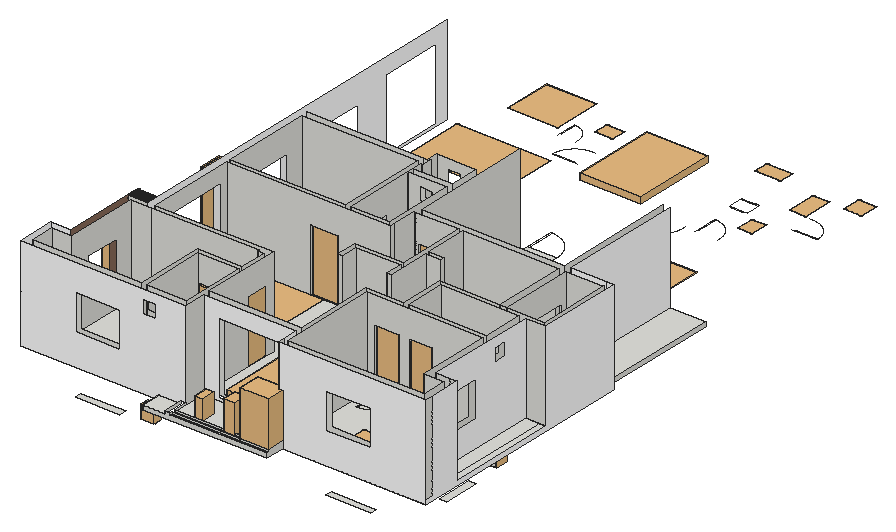
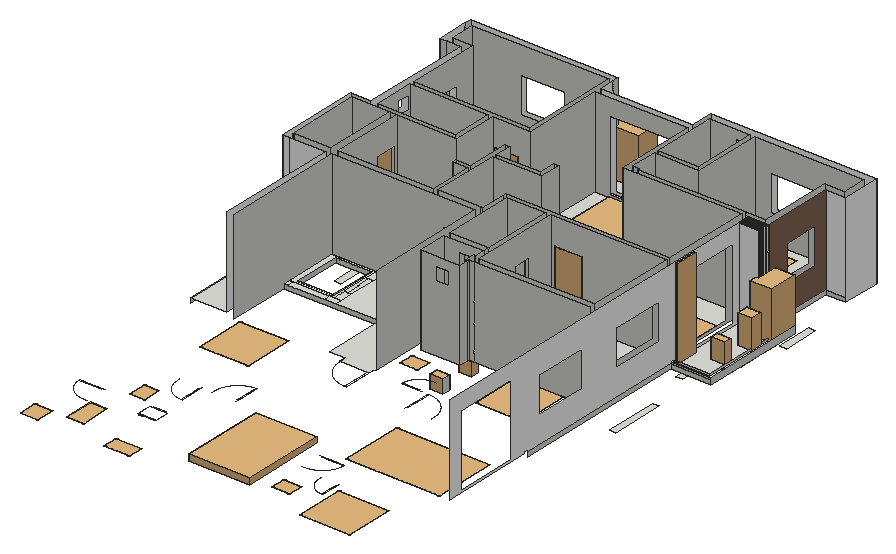
# SketchUp Ruby script. Lengths in inches.
U = 1.inch
M = Sketchup.active_model
def pt(a) = Geom::Point3d.new(a.map { |v| v * U })
def face(e, loops, mat)
  f = e.add_face(loops[0].map { |a| pt(a) })
  loops[1..].each { |l| e.add_face(l.map { |a| pt(a) }).erase! }
  f.material = f.back_material = mat if mat
  f
end
# faces: each face lists its corners as indices into pts; further lists are holes
def faces(e, pts, list, mat = nil) = list.each { |f| face(e, (f[0].is_a?(Array) ? f : [f]).map { |l| l.map { |i| pts[i] } }, mat) }
# xy, xz, yz: faces in a plane at the given z, y or x. An outline is a flat list of corners, or four numbers for a rectangle; further outlines are holes
def ring(l) = l.size == 4 ? [[l[0], l[1]], [l[2], l[1]], [l[2], l[3]], [l[0], l[3]]] : l.each_slice(2).to_a
def flat(e, list, mat, &to3) = list.each { |f| face(e, (f[0].is_a?(Array) ? f : [f]).map { |l| ring(l).map { |u, v| to3.(u, v) } }, mat) }
def xy(e, z, list, mat = nil) = flat(e, list, mat) { |x, y| [x, y, z] }
def xz(e, y, list, mat = nil) = flat(e, list, mat) { |x, z| [x, y, z] }
def yz(e, x, list, mat = nil) = flat(e, list, mat) { |y, z| [x, y, z] }
def lines(e, pts, list) = list.each { |a, b| e.add_line(pt(pts[a]), pt(pts[b])) }
# prism: a flat outline (further loops are holes) pulled along v
def prism(e, loops, v, mat = nil)
  f = face(e, loops, mat); d = Geom::Vector3d.new(v.map { |x| x * U })
  f.pushpull(f.normal.samedirection?(d) ? d.length : -d.length)
end
def box(e, o, s, mat = nil) = prism(e, [[o, [o[0] + s[0], o[1], o[2]], [o[0] + s[0], o[1] + s[1], o[2]], [o[0], o[1] + s[1], o[2]]]], [0, 0, s[2]], mat)
def at(x, y, z, deg = 0) = Geom::Transformation.translation(pt([x, y, z])) * Geom::Transformation.rotation(ORIGIN, Z_AXIS, deg.degrees)
def axes(o, x, y, z) = Geom::Transformation.new([*x, 0, *y, 0, *z, 0, *pt(o).to_a, 1])
def part(name) = M.definitions.add(name)
# library, detail: a bought-in or finely detailed component or shape, given as its bounding box
def library(name, o, s) = part(name).tap { |d| box(d.entities, o, s) }
def detail(e, o, s) = box(e.add_group.entities, o, s)
def put(e, d, t, mat = nil) = e.add_instance(d, t).tap { |i| i.material = mat if mat }
def group(e, t, mat = nil) = e.add_group.tap { |g| g.transformation = t; g.material = mat if mat }.entities
root = M.entities
M.materials.add("Manhattan Creative Coating ML 1016B 24.75cm").color = [255, 255, 255]
M.materials.add("Wintan - wpa36452 29.79cm").color = [255, 255, 255]
M.materials.add("Wood Planks C01 100cm").color = [136, 107, 89]
c1 = library("Potted Plant 02",[-16.98,-19.78,0],[30.04,38.68,37.52])
c2 = library("Potted Plant 13",[-10,-7.28,0],[18.93,15.17,39.22])
c3 = library("Potted Plant 50-12",[-6.11,-5.26,0],[11.24,10.56,13.41])
c4 = library("Window Crafter Awning 2",[0,-9.5,0],[17.5,11.27,18])
c5 = library("Door 243 053",[-21.6,-2.79,-0.07],[43.2,5.58,82.64])
c6 = part("Rectangular column")
box(c6.entities,[0,16,0],[27,1,119.8])
box(c6.entities,[0,3.56,0],[27,1,120])
box(c6.entities,[0,1.78,0],[27,1,120])
box(c6.entities,[0,14.22,0],[27,1,119.8])
box(c6.entities,[0,5.33,0],[27,1,120])
box(c6.entities,[0,7.11,0],[27,1,120])
box(c6.entities,[0,10.67,0],[27,1,120.2])
box(c6.entities,[0,12.44,0],[27,1,119.8])
box(c6.entities,[0,0,0],[27,1,120])
xy(c6.entities,0,[[0,8.89,27,9.89]])
xy(c6.entities,120,[[0,8.89,27,9.89]])
xz(c6.entities,8.89,[[0,0,27,120]])
xz(c6.entities,9.89,[[0,0,27,120]])
yz(c6.entities,0,[[8.89,0,9.89,120]],"Wintan - wpa36452 29.79cm")
yz(c6.entities,27,[[8.89,0,9.89,120]])
c7 = library("Tlon Light 650 Ceiling 152 007",[-12.8,-12.8,-3.78],[25.6,25.6,3.58])
c8 = part("Square rail bar")
box(c8.entities,[0,0,-1],[51.7,1,1])
c9 = part("Group\#20")
xy(c9.entities,0,[[0,0,51.7,106.6]])
xy(c9.entities,1,[[0,0,51.7,107.6]])
xz(c9.entities,0,[[0,0,51.7,1]])
xz(c9.entities,107.6,[[0,0,51.7,1]])
yz(c9.entities,0,[[0,0,107.6,1]])
yz(c9.entities,51.7,[[0,0,107.6,1]])
put(c9.entities,c8,at(0,106.6,0))
put(c9.entities,c8,at(0,0,0))
put(c9.entities,c8,at(0,103.05,0))
put(c9.entities,c8,at(0,99.49,0))
put(c9.entities,c8,at(0,95.94,0))
put(c9.entities,c8,at(0,92.39,0))
put(c9.entities,c8,at(0,88.83,0))
put(c9.entities,c8,at(0,85.28,0))
put(c9.entities,c8,at(0,81.73,0))
put(c9.entities,c8,at(0,78.17,0))
put(c9.entities,c8,at(0,74.62,0))
put(c9.entities,c8,at(0,71.07,0))
put(c9.entities,c8,at(0,67.51,0))
put(c9.entities,c8,at(0,63.96,0))
put(c9.entities,c8,at(0,60.41,0))
put(c9.entities,c8,at(0,56.85,0))
put(c9.entities,c8,at(0,53.3,0))
put(c9.entities,c8,at(0,49.75,0))
put(c9.entities,c8,at(0,46.19,0))
put(c9.entities,c8,at(0,42.64,0))
put(c9.entities,c8,at(0,39.09,0))
put(c9.entities,c8,at(0,35.53,0))
put(c9.entities,c8,at(0,31.98,0))
put(c9.entities,c8,at(0,28.43,0))
put(c9.entities,c8,at(0,24.875,0))
put(c9.entities,c8,at(0,21.32,0))
put(c9.entities,c8,at(0,17.77,0))
put(c9.entities,c8,at(0,14.21,0))
put(c9.entities,c8,at(0,10.66,0))
put(c9.entities,c8,at(0,7.11,0))
put(c9.entities,c8,at(0,3.55,0))
put(c9.entities,c8,at(0,0,0))
c10 = library("Group1606\#2",[0.89,0.19,0],[2.1,4.18,2.5])
c11 = library("A$C403C54AD\#3",[0,0,-0.17],[8.08,5.86,0.57])
c12 = library("TARJA2\#3",[-2.49,-4.93,0],[8.71,4.91,0.01])
c13 = part("A$C42203764\#3")
put(c13.entities,c12,axes([263.32,520.21,0],[105.57605,0,0],[0,105.57605,0],[0,0,105.57605]))
c14 = library("A$C038F079D\#3",[0,0,0],[750,440,0.01])
c15 = library("A$C00C51FE0\#3",[0,0,0],[20,24.125,0.01])
c16 = library("A$C20C229D7\#3",[0,576,0],[24,24,0.01])
c17 = part("A$C659B0DF6\#3")
p = [[21.05,606.07,0],[21.05,607.55,0],[17.35,607.55,0],[17.35,606.07,0],[24,604.22,0],[0,604.22,0],
  [24,606.07,0],[0,606.07,0],[20.625,583.91,0],[20.625,585.72,0],[3.375,583.91,0],[3.375,585.72,0],
  [0,585.72,0],[24,585.72,0]]
lines(c17.entities,p,[[0,1],[2,3],[1,2],[4,5],[6,7],[8,9],[10,11],[10,8],[12,7],[13,6],[13,12]])
c18 = library("A$C4DC51D13\#3",[-0.71,0,0],[4438.2,2996.1875,0.01])
c19 = library("A$C52B64FF5\#3",[0,0,0],[6.95,7.1875,0.01])
c20 = part("*U13\#3")
p = [[0,0,0],[0,24,0],[-1.75,24,0],[-1.75,0,0],[-1.57,23.95,0],[-3.13,23.79,0],
  [-4.68,23.54,0],[-6.21,23.18,0],[-7.71,22.73,0],[-9.18,22.17,0],[-10.61,21.52,0],[-12,20.78,0],
  [-13.33,19.96,0],[-14.61,19.04,0],[-15.82,18.04,0],[-16.97,16.97,0],[-18.04,15.82,0],[-19.04,14.61,0],
  [-19.96,13.33,0],[-20.78,12,0],[-21.52,10.61,0],[-22.17,9.18,0],[-22.73,7.71,0],[-23.18,6.21,0],
  [-23.54,4.68,0],[-23.79,3.13,0],[-23.95,1.57,0],[-24,0,0],[0,-4,0],[-24,-4,0]]
lines(c20.entities,p,[[0,1],[1,2],[2,3],[3,0],[1,4],[4,5],[5,6],[6,7],[7,8],[8,9],[9,10],[10,11],
  [11,12],[12,13],[13,14],[14,15],[15,16],[16,17],[17,18],[18,19],[19,20],[20,21],[21,22],[22,23],
  [23,24],[24,25],[25,26],[26,27],[0,28],[27,29]])
c21 = part("*U14\#3")
p = [[0,0,0],[0,24,0],[1.75,24,0],[1.75,0,0],[24,0,0],[23.95,1.51,0],
  [23.8125,3.01,0],[23.57,4.5,0],[23.25,5.97,0],[22.83,7.42,0],[22.31,8.83,0],[21.72,10.22,0],
  [21.03,11.5625,0],[20.26,12.86,0],[19.42,14.11,0],[18.49,15.3,0],[17.5,16.43,0],[16.43,17.5,0],
  [15.3,18.49,0],[14.11,19.42,0],[12.86,20.26,0],[11.5625,21.03,0],[10.22,21.72,0],[8.83,22.31,0],
  [7.42,22.83,0],[5.97,23.25,0],[4.5,23.57,0],[3.01,23.8125,0],[1.51,23.95,0],[0,-4,0],
  [24,-4,0]]
lines(c21.entities,p,[[0,1],[1,2],[2,3],[3,0],[4,5],[5,6],[6,7],[7,8],[8,9],[9,10],[10,11],[11,12],
  [12,13],[13,14],[14,15],[15,16],[16,17],[17,18],[18,19],[19,20],[20,21],[21,22],[22,23],[23,24],
  [24,25],[25,26],[26,27],[27,28],[28,1],[0,29],[4,30]])
c22 = part("*U15\#3")
p = [[0,0,0],[0,30,0],[-1.75,30,0],[-1.75,0,0],[-1.96,29.9375,0],[-3.92,29.74,0],
  [-5.85,29.42,0],[-7.76,28.98,0],[-9.64,28.41,0],[-11.48,27.72,0],[-13.27,26.91,0],[-15,25.98,0],
  [-16.67,24.94,0],[-18.26,23.8,0],[-19.78,22.56,0],[-21.21,21.21,0],[-22.56,19.78,0],[-23.8,18.26,0],
  [-24.94,16.67,0],[-25.98,15,0],[-26.91,13.27,0],[-27.72,11.48,0],[-28.41,9.64,0],[-28.98,7.76,0],
  [-29.42,5.85,0],[-29.74,3.92,0],[-29.9375,1.96,0],[-30,0,0],[0,-4,0],[-30,-4,0]]
lines(c22.entities,p,[[0,1],[1,2],[2,3],[3,0],[1,4],[4,5],[5,6],[6,7],[7,8],[8,9],[9,10],[10,11],
  [11,12],[12,13],[13,14],[14,15],[15,16],[16,17],[17,18],[18,19],[19,20],[20,21],[21,22],[22,23],
  [23,24],[24,25],[25,26],[26,27],[0,28],[27,29]])
c23 = part("*U12\#3")
p = [[0,0,0],[0,-30,0],[-1.75,-30,0],[-1.75,0,0],[-30,0,0],[-29.94,-1.88,0],
  [-29.76,-3.76,0],[-29.47,-5.62,0],[-29.06,-7.46,0],[-28.53,-9.27,0],[-27.89,-11.04,0],[-27.14,-12.77,0],
  [-26.29,-14.45,0],[-25.33,-16.07,0],[-24.27,-17.63,0],[-23.12,-19.12,0],[-21.87,-20.54,0],[-20.54,-21.87,0],
  [-19.12,-23.12,0],[-17.63,-24.27,0],[-16.07,-25.33,0],[-14.45,-26.29,0],[-12.77,-27.14,0],[-11.04,-27.89,0],
  [-9.27,-28.53,0],[-7.46,-29.06,0],[-5.62,-29.47,0],[-3.76,-29.76,0],[-1.88,-29.94,0],[0,4,0],
  [-30,4,0]]
lines(c23.entities,p,[[0,1],[1,2],[2,3],[3,0],[4,5],[5,6],[6,7],[7,8],[8,9],[9,10],[10,11],[11,12],
  [12,13],[13,14],[14,15],[15,16],[16,17],[17,18],[18,19],[19,20],[20,21],[21,22],[22,23],[23,24],
  [24,25],[25,26],[26,27],[27,28],[28,1],[0,29],[4,30]])
c24 = part("*U9\#3")
p = [[0,0,0],[0,36,0],[-1.75,36,0],[-1.75,0,0],[-2.35,35.92,0],[-4.7,35.69,0],
  [-7.02,35.31,0],[-9.32,34.77,0],[-11.57,34.09,0],[-13.78,33.26,0],[-15.92,32.29,0],[-18,31.18,0],
  [-20,29.93,0],[-21.92,28.5625,0],[-23.74,27.07,0],[-25.46,25.46,0],[-27.07,23.74,0],[-28.5625,21.92,0],
  [-29.93,20,0],[-31.18,18,0],[-32.29,15.92,0],[-33.26,13.78,0],[-34.09,11.57,0],[-34.77,9.32,0],
  [-35.31,7.02,0],[-35.69,4.7,0],[-35.92,2.35,0],[-36,0,0],[0,-4,0],[-36,-4,0]]
lines(c24.entities,p,[[0,1],[1,2],[2,3],[3,0],[1,4],[4,5],[5,6],[6,7],[7,8],[8,9],[9,10],[10,11],
  [11,12],[12,13],[13,14],[14,15],[15,16],[16,17],[17,18],[18,19],[19,20],[20,21],[21,22],[22,23],
  [23,24],[24,25],[25,26],[26,27],[0,28],[27,29]])
c25 = part("*U8\#3")
p = [[0,0,0],[0,-36,0],[-1.75,-36,0],[-1.75,0,0],[-36,0,0],[-35.93,-2.26,0],
  [-35.72,-4.51,0],[-35.36,-6.75,0],[-34.87,-8.95,0],[-34.24,-11.125,0],[-33.47,-13.25,0],[-32.57,-15.33,0],
  [-31.55,-17.34,0],[-30.4,-19.29,0],[-29.125,-21.16,0],[-27.74,-22.95,0],[-26.24,-24.64,0],[-24.64,-26.24,0],
  [-22.95,-27.74,0],[-21.16,-29.125,0],[-19.29,-30.4,0],[-17.34,-31.55,0],[-15.33,-32.57,0],[-13.25,-33.47,0],
  [-11.125,-34.24,0],[-8.95,-34.87,0],[-6.75,-35.36,0],[-4.51,-35.72,0],[-2.26,-35.93,0],[0,4,0],
  [-36,4,0]]
lines(c25.entities,p,[[0,1],[1,2],[2,3],[3,0],[4,5],[5,6],[6,7],[7,8],[8,9],[9,10],[10,11],[11,12],
  [12,13],[13,14],[14,15],[15,16],[16,17],[17,18],[18,19],[19,20],[20,21],[21,22],[22,23],[23,24],
  [24,25],[25,26],[26,27],[27,28],[28,1],[0,29],[4,30]])
c26 = part("*U7\#3")
p = [[0,0,0],[0,24,0],[1.75,24,0],[1.75,0,0],[24,0,0],[23.95,1.51,0],
  [23.8125,3.01,0],[23.57,4.5,0],[23.25,5.97,0],[22.83,7.42,0],[22.31,8.83,0],[21.72,10.22,0],
  [21.03,11.5625,0],[20.26,12.86,0],[19.42,14.11,0],[18.49,15.3,0],[17.5,16.43,0],[16.43,17.5,0],
  [15.3,18.49,0],[14.11,19.42,0],[12.86,20.26,0],[11.5625,21.03,0],[10.22,21.72,0],[8.83,22.31,0],
  [7.42,22.83,0],[5.97,23.25,0],[4.5,23.57,0],[3.01,23.8125,0],[1.51,23.95,0],[0,-4,0],
  [24,-4,0]]
lines(c26.entities,p,[[0,1],[1,2],[2,3],[3,0],[4,5],[5,6],[6,7],[7,8],[8,9],[9,10],[10,11],[11,12],
  [12,13],[13,14],[14,15],[15,16],[16,17],[17,18],[18,19],[19,20],[20,21],[21,22],[22,23],[23,24],
  [24,25],[25,26],[26,27],[27,28],[28,1],[0,29],[4,30]])
c27 = part("*U6\#3")
p = [[0,0,0],[0,-24,0],[1.75,-24,0],[1.75,0,0],[1.51,-23.95,0],[3.01,-23.8125,0],
  [4.5,-23.57,0],[5.97,-23.25,0],[7.42,-22.83,0],[8.83,-22.31,0],[10.22,-21.72,0],[11.5625,-21.03,0],
  [12.86,-20.26,0],[14.11,-19.42,0],[15.3,-18.49,0],[16.43,-17.5,0],[17.5,-16.43,0],[18.49,-15.3,0],
  [19.42,-14.11,0],[20.26,-12.86,0],[21.03,-11.5625,0],[21.72,-10.22,0],[22.31,-8.83,0],[22.83,-7.42,0],
  [23.25,-5.97,0],[23.57,-4.5,0],[23.8125,-3.01,0],[23.95,-1.51,0],[24,0,0],[0,4,0],
  [24,4,0]]
lines(c27.entities,p,[[0,1],[1,2],[2,3],[3,0],[1,4],[4,5],[5,6],[6,7],[7,8],[8,9],[9,10],[10,11],
  [11,12],[12,13],[13,14],[14,15],[15,16],[16,17],[17,18],[18,19],[19,20],[20,21],[21,22],[22,23],
  [23,24],[24,25],[25,26],[26,27],[27,28],[0,29],[28,30]])
c28 = part("*U5\#3")
p = [[0,0,0],[0,-28,0],[1.75,-28,0],[1.75,0,0],[1.76,-27.94,0],[3.51,-27.78,0],
  [5.25,-27.5,0],[6.96,-27.12,0],[8.65,-26.63,0],[10.31,-26.03,0],[11.92,-25.34,0],[13.49,-24.54,0],
  [15,-23.64,0],[16.46,-22.65,0],[17.85,-21.57,0],[19.17,-20.41,0],[20.41,-19.17,0],[21.57,-17.85,0],
  [22.65,-16.46,0],[23.64,-15,0],[24.54,-13.49,0],[25.34,-11.92,0],[26.03,-10.31,0],[26.63,-8.65,0],
  [27.12,-6.96,0],[27.5,-5.25,0],[27.78,-3.51,0],[27.94,-1.76,0],[28,0,0],[0,4,0],
  [28,4,0]]
lines(c28.entities,p,[[0,1],[1,2],[2,3],[3,0],[1,4],[4,5],[5,6],[6,7],[7,8],[8,9],[9,10],[10,11],
  [11,12],[12,13],[13,14],[14,15],[15,16],[16,17],[17,18],[18,19],[19,20],[20,21],[21,22],[22,23],
  [23,24],[24,25],[25,26],[26,27],[27,28],[0,29],[28,30]])
c29 = part("*U4\#3")
p = [[0,0,0],[0,28,0],[1.75,28,0],[1.75,0,0],[28,0,0],[27.94,1.76,0],
  [27.78,3.51,0],[27.5,5.25,0],[27.12,6.96,0],[26.63,8.65,0],[26.03,10.31,0],[25.34,11.92,0],
  [24.54,13.49,0],[23.64,15,0],[22.65,16.46,0],[21.57,17.85,0],[20.41,19.17,0],[19.17,20.41,0],
  [17.85,21.57,0],[16.46,22.65,0],[15,23.64,0],[13.49,24.54,0],[11.92,25.34,0],[10.31,26.03,0],
  [8.65,26.63,0],[6.96,27.12,0],[5.25,27.5,0],[3.51,27.78,0],[1.76,27.94,0],[0,-4,0],
  [28,-4,0]]
lines(c29.entities,p,[[0,1],[1,2],[2,3],[3,0],[4,5],[5,6],[6,7],[7,8],[8,9],[9,10],[10,11],[11,12],
  [12,13],[13,14],[14,15],[15,16],[16,17],[17,18],[18,19],[19,20],[20,21],[21,22],[22,23],[23,24],
  [24,25],[25,26],[26,27],[27,28],[28,1],[0,29],[4,30]])
c30 = part("*U3\#3")
p = [[0,0,0],[0,30,0],[1.75,30,0],[1.75,0,0],[30,0,0],[29.94,1.88,0],
  [29.76,3.76,0],[29.47,5.62,0],[29.06,7.46,0],[28.53,9.27,0],[27.89,11.04,0],[27.14,12.77,0],
  [26.29,14.45,0],[25.33,16.07,0],[24.27,17.63,0],[23.12,19.12,0],[21.87,20.54,0],[20.54,21.87,0],
  [19.12,23.12,0],[17.63,24.27,0],[16.07,25.33,0],[14.45,26.29,0],[12.77,27.14,0],[11.04,27.89,0],
  [9.27,28.53,0],[7.46,29.06,0],[5.62,29.47,0],[3.76,29.76,0],[1.88,29.94,0],[0,-4,0],
  [30,-4,0]]
lines(c30.entities,p,[[0,1],[1,2],[2,3],[3,0],[4,5],[5,6],[6,7],[7,8],[8,9],[9,10],[10,11],[11,12],
  [12,13],[13,14],[14,15],[15,16],[16,17],[17,18],[18,19],[19,20],[20,21],[21,22],[22,23],[23,24],
  [24,25],[25,26],[26,27],[27,28],[28,1],[0,29],[4,30]])
c31 = part("*U2\#3")
p = [[0,0,0],[0,-32,0],[1.75,-32,0],[1.75,0,0],[2.01,-31.9375,0],[4.01,-31.75,0],
  [6,-31.43,0],[7.96,-30.99,0],[9.89,-30.43,0],[11.78,-29.75,0],[13.625,-28.95,0],[15.42,-28.04,0],
  [17.15,-27.02,0],[18.81,-25.89,0],[20.4,-24.66,0],[21.91,-23.33,0],[23.33,-21.91,0],[24.66,-20.4,0],
  [25.89,-18.81,0],[27.02,-17.15,0],[28.04,-15.42,0],[28.95,-13.625,0],[29.75,-11.78,0],[30.43,-9.89,0],
  [30.99,-7.96,0],[31.43,-6,0],[31.75,-4.01,0],[31.9375,-2.01,0],[32,0,0],[0,4,0],
  [32,4,0]]
lines(c31.entities,p,[[0,1],[1,2],[2,3],[3,0],[1,4],[4,5],[5,6],[6,7],[7,8],[8,9],[9,10],[10,11],
  [11,12],[12,13],[13,14],[14,15],[15,16],[16,17],[17,18],[18,19],[19,20],[20,21],[21,22],[22,23],
  [23,24],[24,25],[25,26],[26,27],[27,28],[0,29],[28,30]])
c32 = part("Commercial Building Flr Plans.dwg\#3")
xy(c32.entities,0,[[722.01,373.53,728.01,373.53,728.01,396.03,788.01,396.03,788.01,373.53,794.01,373.53,794.01,430.53,814.01,430.53,814.01,436.53,794.01,436.53,794.01,493.53,923.01,493.53,923.01,487.53,932.01,487.53,932.01,493.53,918.01,493.53,918.01,502.53,868.01,502.53,868.01,493.53,854.01,493.53,854.01,502.53,773.01,502.53,773.01,493.53,788.01,493.53,788.01,502.53,802.01,502.53,802.01,493.53,788.01,493.53,788.01,402.03,722.01,402.03],[854.01,493.53,868.01,502.53],[918.01,493.53,932.01,502.53],[854.01,502.53,863.01,520.53],[[863.01,502.53,923.01,574.53],[867.01,506.53,915.01,570.53]],
  [923.01,502.53,932.01,502.53,932.01,583.53,932.01,574.53,923.01,574.53],[854.01,520.53,859.01,520.53,859.01,538.53,858.01,538.53,858.01,556.53,854.01,556.53],[859.01,520.53,860.01,538.53],[860.01,520.53,863.01,520.53,863.01,556.53,859.01,556.53,859.01,538.53,860.01,538.53],[858.01,538.53,859.01,556.53],
  [854.01,556.53,863.01,574.53],[854.01,574.53,868.01,583.53],[918.01,574.53,932.01,583.53]])
xz(c32.entities,506.53,[[867.01,-6,915.01,0]])
xz(c32.entities,570.53,[[867.01,-6,915.01,0]])
yz(c32.entities,867.01,[[506.53,-6,570.53,0]])
yz(c32.entities,915.01,[[506.53,-6,570.53,0]])
# 5414 loose lines left out
put(c32.entities,c11,axes([684.95,938.32,0.02],[0,-14.03023,0],[14.03023,0,0],[0,0,14.03023]))
put(c32.entities,c11,axes([684.95,346.29,0.02],[0,-14.03023,0],[14.03023,0,0],[0,0,14.03023]))
put(c32.entities,c13,axes([900.04,908.53,0],[0,0.04349,0],[0.04349,0,0],[0,0,0.04349]))
put(c32.entities,c13,axes([900.04,428.53,0],[0,0.04349,0],[0.04349,0,0],[0,0,0.04349]))
put(c32.entities,c14,axes([819.23,471.91,0],[0.04545,0,0],[0,0.04545,0],[0,0,0.04545]))
put(c32.entities,c14,axes([819.23,951.91,0],[0.04545,0,0],[0,0.04545,0],[0,0,0.04545]))
put(c32.entities,c15,axes([722.01,550.53,0],[0,-1,0],[-1,0,0],[0,0,1]))
put(c32.entities,c15,at(660.51,238.53,0,90))
put(c32.entities,c15,at(722.01,619.53,0,90))
put(c32.entities,c15,at(660.51,911.53,0,90))
put(c32.entities,c15,at(901.51,868.5,0,180))
put(c32.entities,c15,at(904.51,388.5,0,180))
put(c32.entities,c16,at(942.55,371.21,0))
put(c32.entities,c16,at(945.55,-108.79,0))
put(c32.entities,c17,at(845.01,-189.39,0))
put(c32.entities,c17,at(845.01,290.61,0))
put(c32.entities,c18,axes([512.64,369.84,0],[0.02827,0,0],[0,0.02827,0],[0,0,0.02827]))
put(c32.entities,c18,axes([512.64,750.84,0],[0.02827,0,0],[0,0.02827,0],[0,0,0.02827]))
put(c32.entities,c19,axes([533.03,959.68,0],[0,-9.39007,0],[9.39007,0,0],[0,0,9.39007]))
put(c32.entities,c19,axes([841.85,744,0],[9.39007,0,0],[0,-9.39007,0],[0,0,9.39007]))
put(c32.entities,c19,axes([844.85,264,0],[9.39007,0,0],[0,-9.39007,0],[0,0,9.39007]))
put(c32.entities,c19,axes([541.85,657,0],[9.39007,0,0],[0,-9.39007,0],[0,0,9.39007]))
put(c32.entities,c19,axes([541.85,513.06,0],[9.39007,0,0],[0,9.39007,0],[0,0,9.39007]))
put(c32.entities,c19,axes([533.03,275.68,0],[0,-9.39007,0],[9.39007,0,0],[0,0,9.39007]))
put(c32.entities,c20,at(669.51,496.53,0,-90))
put(c32.entities,c21,at(669.51,673.53,0,-90))
put(c32.entities,c22,at(932.01,397.53,0,-90))
put(c32.entities,c22,at(932.01,877.53,0,-90))
put(c32.entities,c23,at(660.51,292.53,0,-90))
put(c32.entities,c23,at(660.51,847.03,0,-90))
put(c32.entities,c24,at(657.51,460.53,0))
put(c32.entities,c25,at(657.51,709.53,0))
put(c32.entities,c26,at(609.51,886.53,0))
put(c32.entities,c27,at(609.51,283.53,0))
put(c32.entities,c28,axes([734.01,493.53,0],[1.39286,0,0],[0,1.39286,0],[0,0,1.39286]))
put(c32.entities,c29,axes([734.01,676.53,0],[1.39286,0,0],[0,1.39286,0],[0,0,1.39286]))
put(c32.entities,c30,at(854.01,334.53,0))
put(c32.entities,c30,at(851.01,814.53,0))
put(c32.entities,c31,at(807.51,328.53,0))
put(c32.entities,c31,at(804.51,808.53,0))
xy(root,336,[[1863.02,500.67,1923.02,509.67],[2199.52,500.67,2259.52,509.67],[1816.02,569.57,1825.02,617.57],[2297.52,569.57,2306.52,617.57],[1954.02,596.67,1978.02,602.67],
  [2005.02,605.67,2011.02,635.67],[2152.02,641.67,2184.02,647.67],[2198.52,641.67,2228.52,647.67],[2267.52,710.67,2276.52,740.67],[2267.52,752.67,2276.52,800.67],
  [1966.02,767.67,2002.02,773.67],[1843.02,797.67,1852.02,869.67],[2078.52,806.67,2117.52,815.67],[2008.02,809.67,2014.02,833.67]])
xy(root,342,[[1953.02,500.67,1970.52,509.67],[2297.52,649.73,2306.52,667.23],[2029.77,869.67,2047.27,878.67]])
xy(root,351,[[2031.27,530.62,2115.27,539.67],[1843.02,673.67,1852.02,757.67]])
xy(root,360,[[1953.02,500.67,1970.52,509.67],[2297.52,649.73,2306.52,667.23],[2029.77,869.67,2047.27,878.67],[2029.77,917.67,2047.27,926.67]])
xy(root,372,[[[2135.52,500.67,2333.52,500.67,2333.52,551.67,2306.52,551.67,2306.52,701.67,2333.52,701.67,2333.52,806.67,2327.52,806.67,2327.52,707.67,2186.52,707.67,2186.52,647.67,2135.52,647.67,2135.52,539.67,2011.02,539.67,2011.02,530.62,2135.52,530.62],[2141.52,509.67,2141.52,641.67,2297.52,641.67,2297.52,542.67,2324.52,542.67,2324.52,509.67],[2192.52,647.67,2297.52,701.67]],[1945.02,509.67,1951.02,509.67,1951.02,596.67,2005.02,596.67,2005.02,602.67,1945.02,602.67],[2267.52,707.67,2276.52,806.67],[2324.52,806.67,2333.52,815.67],[2014.02,869.67,2066.52,878.67]])
xy(root,378,[[1975.05,473.67,2005.02,500.67],[2011.02,473.67,2141.52,476.67],[2011.02,482.67,2135.52,530.62],[1798.02,509.67,1945.02,509.67,1945.02,602.67,1954.02,602.67,1954.02,596.67,1951.02,596.67,1951.02,509.67,2005.02,509.67,2005.02,596.67,1978.02,596.67,1978.02,602.67,2005.02,602.67,2005.02,605.67,2011.02,605.67,2011.02,635.67,2005.02,635.67,2005.02,638.67,1997.02,638.67,1997.02,641.67,1825.02,641.67,1825.02,542.67,1798.02,542.67],[2141.52,509.67,2324.52,509.67,2324.52,542.67,2297.52,542.67,2297.52,641.67,2228.52,641.67,2228.52,647.67,2198.52,647.67,2198.52,641.67,2184.02,641.67,2184.02,647.67,2152.02,647.67,2152.02,641.67,2141.52,641.67],
  [2011.02,539.67,2135.52,539.67,2135.52,647.67,2186.52,647.67,2186.52,707.67,2267.52,707.67,2267.52,710.67,2276.52,710.67,2276.52,740.67,2267.52,740.67,2267.52,806.67,2138.52,806.67,2138.52,749.67,2158.52,749.67,2158.52,743.67,2138.52,743.67,2138.52,686.67,2132.52,686.67,2132.52,709.17,2072.52,709.17,2072.52,686.67,2066.52,686.67,2066.52,715.17,2132.52,715.17,2132.52,806.67,2117.52,806.67,2117.52,815.67,2078.52,815.67,2078.52,806.67,2072.52,806.67,2072.52,767.67,1852.02,767.67,1852.02,647.67,2011.02,647.67],[2306.52,551.67,2324.52,701.67],[2324.52,551.67,2333.52,701.67],[1795.02,643.17,1816.02,643.17,1816.02,647.67,1843.02,647.67,1843.02,772.17,1795.02,772.17],[2192.52,647.67,2297.52,701.67],
  [2066.52,686.67,2072.52,686.67,2072.52,709.17,2132.52,709.17,2132.52,686.67,2138.52,686.67,2138.52,743.67,2158.52,743.67,2158.52,749.67,2138.52,749.67,2138.52,806.67,2132.52,806.67,2132.52,715.17,2066.52,715.17],[2276.52,707.67,2324.52,806.67],[2324.52,707.67,2327.52,806.67],[1966.02,767.67,2002.02,767.67,2002.02,773.67,2008.02,773.67,2008.02,809.67,2014.02,809.67,2014.02,833.67,2008.02,833.67,2008.02,893.67,1852.02,893.67,1852.02,773.67,1966.02,773.67],[2014.02,773.67,2066.52,869.67],
  [2075.52,815.67,2207.52,815.67,2207.52,887.67,2267.52,887.67,2267.52,896.67,2138.52,896.67,2138.52,980.67,2117.52,980.67,2117.52,989.67,2078.52,989.67,2078.52,980.67,2075.52,980.67],[2276.52,815.67,2324.52,980.67],[2014.02,878.67,2066.52,878.67,2066.52,917.67,2014.02,917.67,2014.02,905.17,2017.02,905.17,2017.02,891.17,2014.02,891.17]])
xz(root,473.67,[[1975.05,372,2141.52,372,2141.52,378,2011.02,378,2011.02,381,2005.02,381,2005.02,378,1975.05,378]])
xz(root,476.67,[[2011.02,378,2141.52,381]])
xz(root,482.67,[[2011.02,378,2135.52,381]])
xz(root,500.67,[[[1789.02,372,1975.05,372,1975.05,378,2005.02,378,2005.02,381,2011.02,381,2011.02,498,1789.02,498],[1863.02,414,1923.02,462],[1953.02,468,1970.52,486]],[[2141.52,372,2333.52,372,2333.52,498,2135.52,498,2135.52,381,2141.52,381],[2199.52,414,2259.52,462]]],"Manhattan Creative Coating ML 1016B 24.75cm")
xz(root,509.67,[[[1798.02,378,1945.02,498],[1863.02,414,1923.02,462]],[[1951.02,378,2005.02,498],[1953.02,468,1970.52,486]],[[2141.52,378,2324.52,498],[2199.52,414,2259.52,462]]])
xz(root,530.62,[[[2011.02,378,2135.52,498],[2031.27,381,2115.27,477]]],"Manhattan Creative Coating ML 1016B 24.75cm")
xz(root,539.67,[[[2011.02,378,2135.52,498],[2031.27,381,2115.27,477]]])
xz(root,542.67,[[1798.02,378,1825.02,498],[2297.52,378,2324.52,498]])
xz(root,551.67,[[1789.02,372,1816.02,378],[2306.52,378,2324.52,498],[2324.52,378,2333.52,498]])
xz(root,551.67,[[1789.02,378,1816.02,498]],"Manhattan Creative Coating ML 1016B 24.75cm")
xz(root,596.67,[[1951.02,378,1954.02,378,1954.02,462,1978.02,462,1978.02,378,2005.02,378,2005.02,498,1951.02,498]])
xz(root,602.67,[[1945.02,378,1945.02,498,2005.02,498,2005.02,378,1978.02,378,1978.02,462,1954.02,462,1954.02,378]])
xz(root,605.67,[[2005.02,378,2011.02,462]])
xz(root,635.67,[[2005.02,378,2011.02,462]])
xz(root,637.17,[[1789.02,372,1816.02,378],[1789.02,378,1816.02,381]])
xz(root,638.67,[[1997.02,378,2005.02,498]])
xz(root,641.67,[[1825.02,378,1852.02,498],[1852.02,378,1997.02,498],[2141.52,378,2152.02,378,2152.02,462,2184.02,462,2184.02,378,2198.52,378,2198.52,462,2228.52,462,2228.52,378,2297.52,378,2297.52,498,2141.52,498]])
xz(root,643.17,[[1795.02,378,1816.02,381]])
xz(root,647.67,[[1816.02,378,1843.02,498],[1852.02,378,2011.02,498],[2135.52,378,2135.52,498,2186.52,498,2186.52,378,2184.02,378,2184.02,462,2152.02,462,2152.02,378],[2192.52,378,2192.52,498,2297.52,498,2297.52,378,2228.52,378,2228.52,462,2198.52,462,2198.52,378]])
xz(root,649.73,[[2297.52,342,2306.52,360]])
xz(root,667.23,[[2297.52,342,2306.52,360]])
xz(root,686.67,[[2066.52,378,2072.52,498],[2132.52,378,2138.52,498]])
xz(root,701.67,[[2192.52,378,2297.52,498],[2306.52,378,2333.52,498]])
xz(root,707.67,[[2186.52,378,2267.52,498],[2267.52,378,2276.52,498],[2276.52,378,2327.52,498]])
xz(root,709.17,[[2072.52,378,2132.52,498]])
xz(root,710.67,[[2267.52,378,2276.52,462]])
xz(root,715.17,[[2066.52,378,2132.52,498]])
xz(root,740.67,[[2267.52,378,2276.52,462]])
xz(root,743.67,[[2138.52,378,2158.52,498]])
xz(root,749.67,[[2138.52,378,2158.52,498]])
xz(root,767.67,[[1852.02,378,1966.02,378,1966.02,462,2002.02,462,2002.02,378,2072.52,378,2072.52,498,1852.02,498]])
xz(root,772.17,[[1795.02,378,1843.02,381]])
xz(root,773.67,[[1852.02,378,1852.02,498,2008.02,498,2008.02,378,2002.02,378,2002.02,462,1966.02,462,1966.02,378],[2014.02,378,2066.52,498]])
xz(root,778.17,[[1789.02,372,1843.02,378],[1789.02,378,1843.02,381]])
xz(root,806.67,[[2072.52,378,2075.52,498],[2075.52,378,2078.52,378,2078.52,462,2117.52,462,2117.52,378,2132.52,378,2132.52,498,2075.52,498],[2138.52,378,2267.52,498],[2276.52,378,2324.52,498],[2324.52,378,2327.52,498]])
xz(root,809.67,[[2008.02,378,2014.02,462]])
xz(root,815.67,[[2075.52,378,2075.52,498,2267.52,498,2267.52,378,2117.52,378,2117.52,462,2078.52,462,2078.52,378]])
xz(root,815.67,[[2324.52,372,2333.52,498],[2276.52,378,2324.52,498]],"Manhattan Creative Coating ML 1016B 24.75cm")
xz(root,833.67,[[2008.02,378,2014.02,462]])
xz(root,869.67,[[[2014.02,378,2066.52,498],[2029.77,468,2047.27,486]]])
xz(root,878.67,[[[2014.02,378,2066.52,498],[2029.77,468,2047.27,486]]])
xz(root,891.17,[[2014.02,378,2017.02,498]])
xz(root,893.67,[[1852.02,378,2008.02,498]])
xz(root,896.67,[[2138.52,372,2267.52,378]])
xz(root,902.67,[[1852.02,378,2008.02,498],[2008.02,378,2014.02,498]])
xz(root,905.17,[[2014.02,378,2017.02,498]])
xz(root,917.67,[[[2014.02,378,2066.52,498],[2029.77,468,2047.27,486]]])
yz(root,1789.02,[[637.17,372,778.17,381]])
yz(root,1789.02,[[500.67,372,551.67,498]],"Manhattan Creative Coating ML 1016B 24.75cm")
yz(root,1795.02,[[643.17,378,772.17,381]])
yz(root,1798.02,[[509.67,378,542.67,498]])
yz(root,1816.02,[[551.67,372,637.17,378]])
yz(root,1816.02,[[[551.67,378,551.67,498,647.67,498,647.67,378,643.17,378,643.17,381,637.17,381,637.17,378],[569.57,414,617.57,462]]],"Wood Planks C01 100cm")
yz(root,1825.02,[[[542.67,378,641.67,498],[569.57,414,617.57,462]]])
yz(root,1843.02,[[778.17,372,1018.17,378]])
yz(root,1843.02,[[[647.67,378,647.67,498,1148.67,498,1148.67,378,1024.17,378,1024.17,381,1018.17,381,1018.17,378,778.17,378,778.17,381,772.17,381,772.17,378],[1046.67,381,1130.67,477],[673.67,381,757.67,477],[926.67,414,998.67,462],[797.67,414,869.67,462]]],"Manhattan Creative Coating ML 1016B 24.75cm")
yz(root,1852.02,[[[647.67,378,767.67,498],[673.67,381,757.67,477]],[[773.67,378,893.67,498],[797.67,414,869.67,462]]])
yz(root,1945.02,[[509.67,378,602.67,498]])
yz(root,1951.02,[[509.67,378,596.67,498]])
yz(root,1953.02,[[500.67,342,509.67,360]])
yz(root,1954.02,[[596.67,378,602.67,462]])
yz(root,1966.02,[[767.67,378,773.67,462]])
yz(root,1970.52,[[500.67,342,509.67,360]])
yz(root,1975.05,[[473.67,372,500.67,378]])
yz(root,1978.02,[[596.67,378,602.67,462]])
yz(root,1997.02,[[638.67,378,641.67,498]])
yz(root,2002.02,[[767.67,378,773.67,462]])
yz(root,2005.02,[[473.67,378,500.67,381],[509.67,378,596.67,498],[602.67,378,602.67,498,638.67,498,638.67,378,635.67,378,635.67,462,605.67,462,605.67,378]])
yz(root,2008.02,[[773.67,378,773.67,498,893.67,498,893.67,378,833.67,378,833.67,462,809.67,462,809.67,378]])
yz(root,2011.02,[[473.67,378,476.67,381],[482.67,378,500.67,381],[500.67,378,530.62,498],[539.67,378,605.67,378,605.67,462,635.67,462,635.67,378,647.67,378,647.67,498,539.67,498]])
yz(root,2014.02,[[773.67,378,809.67,378,809.67,462,833.67,462,833.67,378,869.67,378,869.67,498,773.67,498],[869.67,378,878.67,498],[878.67,378,891.17,498],[902.67,378,905.17,498],[905.17,378,917.67,498]])
yz(root,2017.02,[[891.17,378,905.17,498]])
yz(root,2029.77,[[869.67,342,878.67,360],[917.67,342,926.67,360]])
yz(root,2047.27,[[869.67,342,878.67,360],[917.67,342,926.67,360]])
yz(root,2066.52,[[686.67,378,715.17,498],[773.67,378,869.67,498],[878.67,378,917.67,498]])
yz(root,2072.52,[[686.67,378,709.17,498],[767.67,378,773.67,498],[773.67,378,806.67,498]])
yz(root,2075.52,[[815.67,378,980.67,498]])
yz(root,2078.52,[[806.67,378,815.67,462]])
yz(root,2117.52,[[806.67,378,815.67,462]])
yz(root,2132.52,[[686.67,378,709.17,498],[715.17,378,806.67,498]])
yz(root,2135.52,[[482.67,378,500.67,381],[500.67,378,509.67,498],[539.67,378,647.67,498]])
yz(root,2135.52,[[509.67,378,530.62,498]],"Manhattan Creative Coating ML 1016B 24.75cm")
yz(root,2138.52,[[686.67,378,743.67,498],[749.67,378,806.67,498]])
yz(root,2141.52,[[473.67,372,500.67,372,500.67,381,476.67,381,476.67,378,473.67,378],[509.67,378,641.67,498]])
yz(root,2152.02,[[641.67,378,647.67,462]])
yz(root,2158.52,[[743.67,378,749.67,498]])
yz(root,2184.02,[[641.67,378,647.67,462]])
yz(root,2186.52,[[647.67,378,707.67,498]])
yz(root,2192.52,[[647.67,378,701.67,498]])
yz(root,2198.52,[[641.67,378,647.67,462]])
yz(root,2228.52,[[641.67,378,647.67,462]])
yz(root,2267.52,[[896.67,372,896.67,378,815.67,378,815.67,498,980.67,498,980.67,372],[[707.67,378,707.67,498,806.67,498,806.67,378,740.67,378,740.67,462,710.67,462,710.67,378],[752.67,414,800.67,462]]])
yz(root,2276.52,[[[707.67,378,710.67,378,710.67,462,740.67,462,740.67,378,806.67,378,806.67,498,707.67,498],[752.67,414,800.67,462]]])
yz(root,2276.52,[[815.67,378,980.67,498]],"Manhattan Creative Coating ML 1016B 24.75cm")
yz(root,2297.52,[[[542.67,378,641.67,498],[569.57,414,617.57,462]],[[647.67,378,701.67,498],[649.73,468,667.23,486]]])
yz(root,2306.52,[[[551.67,378,701.67,498],[569.57,414,617.57,462],[649.73,468,667.23,486]]],"Manhattan Creative Coating ML 1016B 24.75cm")
yz(root,2324.52,[[815.67,372,980.67,378],[509.67,378,542.67,498]])
yz(root,2327.52,[[707.67,378,806.67,498]])
yz(root,2333.52,[[500.67,378,509.67,498]])
yz(root,2333.52,[[500.67,372,815.67,372,815.67,498,701.67,498,701.67,378,551.67,378,551.67,498,509.67,498,509.67,378,500.67,378]],"Manhattan Creative Coating ML 1016B 24.75cm")
put(root,c1,axes([2121.74,493.66,378],[0,1,0],[-1,0,0],[0,0,1.71]))
put(root,c2,at(2084.22,492.59,378,90))
put(root,c3,axes([2040.7,496.15,378],[0,1.65,0],[-1,0,0],[0,0,2]))
put(root,c4,at(1953.02,507.9,342))
put(root,c5,axes([1965.99,597.61,378],[-0.55696,0,0],[0,-1.07698,0],[0,0,1.01843]))
put(root,c5,axes([2006.02,620.3,378.07],[0,-0.71149,0],[1.07698,0,0],[0,0,1.01843]))
put(root,c5,axes([2213.52,646.74,377.43],[0.69441,0,0],[0,0.74,0],[0,0,1.01843]))
put(root,c5,axes([2168.02,646.74,377.43],[0.7407,0,0],[0,0.74,0],[0,0,1.01843]))
put(root,c6,at(1816.02,647.67,378),"Wintan - wpa36452 29.79cm")
put(root,c1,axes([1806.01,656.95,378],[1,0,0],[0,1,0],[0,0,1.71]))
put(root,c4,at(2299.3,649.73,342,90))
put(root,c7,axes([1817.33,677.24,370.22],[0.44,0,0],[0,0.44,0],[0,0,0.44]))
put(root,c2,at(1804.9375,694.48,378))
put(root,c9,axes([1791.32,664.67,370.98],[1,0,0],[0,0.72,0],[0,0,1]))
put(root,c7,axes([1817.33,723.4375,370.22],[0.44,0,0],[0,0.44,0],[0,0,0.44]))
put(root,c5,axes([2274.59,725.67,378.07],[0,-0.69441,0],[0.74,0,0],[0,0,1.01843]))
put(root,c3,axes([1808.5,738,378],[1.65,0,0],[0,1,0],[0,0,2]))
put(root,c10,axes([1841.02,784.99,372.55],[0,-14.41,0],[0,0,28.70953],[-1,0,0]))
put(root,c5,axes([1984.02,771.84,377.91],[0.83329,0,0],[0,0.74,0],[0,0,1.01843]))
put(root,c5,axes([2097.77,811.09,378.07],[0.9143,0,0],[0,0.74,0],[0,0,1.01843]))
put(root,c4,at(2047.27,869.67,342,180))
put(root,c32,at(1344.52,313.15,378))
put(root,c4,at(2029.77,924.9,342))
